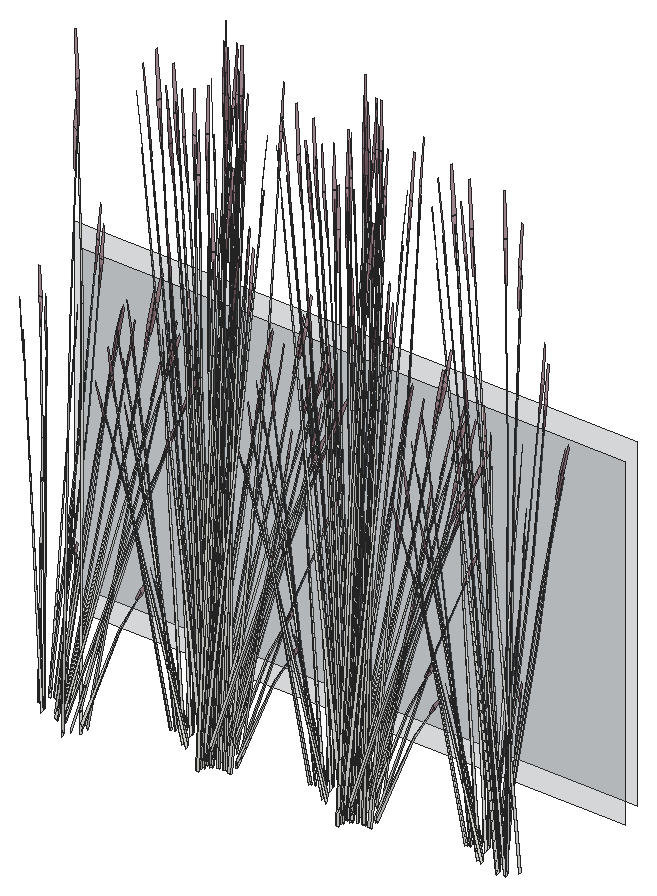
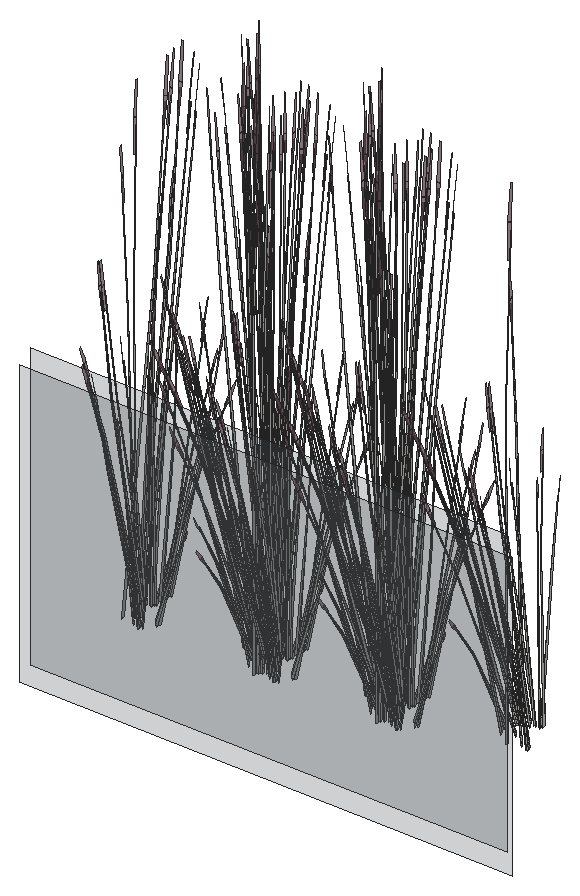
# SketchUp Ruby script. Lengths in inches.
U = 1.inch
M = Sketchup.active_model
def pt(a) = Geom::Point3d.new(a.map { |v| v * U })
def face(e, loops, mat)
  f = e.add_face(loops[0].map { |a| pt(a) })
  loops[1..].each { |l| e.add_face(l.map { |a| pt(a) }).erase! }
  f.material = f.back_material = mat if mat
  f
end
# faces: each face lists its corners as indices into pts; further lists are holes
def faces(e, pts, list, mat = nil) = list.each { |f| face(e, (f[0].is_a?(Array) ? f : [f]).map { |l| l.map { |i| pts[i] } }, mat) }
# xy, xz, yz: faces in a plane at the given z, y or x. An outline is a flat list of corners, or four numbers for a rectangle; further outlines are holes
def ring(l) = l.size == 4 ? [[l[0], l[1]], [l[2], l[1]], [l[2], l[3]], [l[0], l[3]]] : l.each_slice(2).to_a
def flat(e, list, mat, &to3) = list.each { |f| face(e, (f[0].is_a?(Array) ? f : [f]).map { |l| ring(l).map { |u, v| to3.(u, v) } }, mat) }
def xy(e, z, list, mat = nil) = flat(e, list, mat) { |x, y| [x, y, z] }
def xz(e, y, list, mat = nil) = flat(e, list, mat) { |x, z| [x, y, z] }
def yz(e, x, list, mat = nil) = flat(e, list, mat) { |y, z| [x, y, z] }
def lines(e, pts, list) = list.each { |a, b| e.add_line(pt(pts[a]), pt(pts[b])) }
# prism: a flat outline (further loops are holes) pulled along v
def prism(e, loops, v, mat = nil)
  f = face(e, loops, mat); d = Geom::Vector3d.new(v.map { |x| x * U })
  f.pushpull(f.normal.samedirection?(d) ? d.length : -d.length)
end
def box(e, o, s, mat = nil) = prism(e, [[o, [o[0] + s[0], o[1], o[2]], [o[0] + s[0], o[1] + s[1], o[2]], [o[0], o[1] + s[1], o[2]]]], [0, 0, s[2]], mat)
def at(x, y, z, deg = 0) = Geom::Transformation.translation(pt([x, y, z])) * Geom::Transformation.rotation(ORIGIN, Z_AXIS, deg.degrees)
def axes(o, x, y, z) = Geom::Transformation.new([*x, 0, *y, 0, *z, 0, *pt(o).to_a, 1])
def part(name) = M.definitions.add(name)
# library, detail: a bought-in or finely detailed component or shape, given as its bounding box
def library(name, o, s) = part(name).tap { |d| box(d.entities, o, s) }
def detail(e, o, s) = box(e.add_group.entities, o, s)
def put(e, d, t, mat = nil) = e.add_instance(d, t).tap { |i| i.material = mat if mat }
def group(e, t, mat = nil) = e.add_group.tap { |g| g.transformation = t; g.material = mat if mat }.entities
root = M.entities
M.materials.add("Glass_Basic_01").color = [105, 113, 122]
M.materials["Glass_Basic_01"].alpha = 0.25
M.materials.add("LightPink_Translucent").color = [144, 107, 117]
M.materials["LightPink_Translucent"].alpha = 0.75
c1 = part("blade")
p = [[2.15,0.21,22],[0,0.17,0],[0.09,0.45,0],[2.18,0.31,22],[2.29,0.31,22],[0.38,0.45,0],
  [2.48,0.24,33],[2.49,0.24,33],[2.48,0.22,33]]
faces(c1.entities,p,[[0,1,2,3],[4,5,2,3],[6,3,4,7],[8,0,3,6]])
c2 = part("seeds")
p = [[0.3,-0.1,1.38],[-0.01,-0.03,1.59],[-0.01,-0.03,0.03],[0.14,-0.07,-0.07],[0.29,-0.03,3],[0.15,0.01,3.11]]
faces(c2.entities,p,[[0,1,2,3],[1,0,4,5]],"LightPink_Translucent")
c3 = part("blade with seeds")
put(c3.entities,c1,at(0,0,0))
put(c3.entities,c2,axes([2.4,0.25,30.99],[1.5799,-0.05474,1.17369],[-0.12525,1.92788,0.29478],[-0.07173,-0.02425,1.56792]))
xz(root,474,[[218,398,271.49,430]],"Glass_Basic_01")
xz(root,477,[[215,398,270.25,430]],"Glass_Basic_01")
put(root,c3,axes([227.49,457.1,399.875],[0.1255,-0.16547,1.71376],[0.31687,0.44665,0.13857],[-0.21734,0.2034,0.73262]))
put(root,c3,axes([227.39,457.51,399.875],[0.09355,-0.18511,1.71376],[0.39247,0.38307,0.13857],[-0.17705,0.23875,0.73262]))
put(root,c3,axes([227.09,457.59,400.68],[0.12908,0.49174,-0.51099],[-0.48882,0.08602,-0.3958],[-0.14008,0.13208,0.97773]))
put(root,c3,axes([227.34,459.37,398.59],[0.15856,-0.08496,1.43002],[0.39147,0.25616,-0.30754],[-0.11652,0.22165,0.61141]))
put(root,c3,axes([227.5,458.56,400.53],[-0.33997,0.28354,-0.35414],[-0.32182,-0.32376,0.4572],[-0.04897,0.1645,0.87481]))
put(root,c3,axes([227.73,458.26,401.34],[-0.01307,0.49815,-0.7886],[-0.55054,-0.03346,0.09517],[-0.0581,0.21104,1.11556]))
put(root,c3,axes([227.72,459.66,398.77],[-0.013,-0.32022,1.1486],[0.32493,0.22839,0.84392],[-0.0639,0.15263,0.25299]))
put(root,c3,axes([227.54,458.96,399.36],[0.01104,-0.27801,1.54345],[0.49652,0.14685,0.21329],[-0.04302,0.2963,0.72882]))
put(root,c3,axes([227.84,458.42,401],[0.35968,0.36185,-0.5672],[-0.37996,0.3169,-0.43934],[-0.05473,0.18385,1.08528]))
put(root,c3,axes([229.96,456.59,398.84],[-0.01373,-0.50706,1.41272],[0.62119,0.13144,0.59816],[-0.14692,0.27746,1.3335]))
put(root,c3,axes([227.45,458.96,398.82],[0.45645,-0.09537,0.06507],[0.10494,0.38421,-0.86304],[-0.02894,0.19449,0.7736]))
put(root,c3,axes([228.25,457.9,399.875],[-0.0123,-0.2067,1.71376],[0.53301,0.13712,0.13857],[-0.03297,0.29456,0.73262]))
put(root,c3,axes([230.23,458.73,398.375],[0.31414,0.53965,0],[-0.52557,0.30095,-0.51607],[-0.1197,0.06854,1.63711]))
put(root,c3,axes([228.68,459.06,400.53],[-0.15148,0.41415,-0.35414],[-0.44193,-0.12079,0.4572],[0.04052,0.16674,0.87481]))
put(root,c3,axes([228.73,458.68,400.98],[0.23981,0.43789,-0.71045],[-0.49365,0.24404,0.08574],[0.05608,0.21158,1.00501]))
put(root,c3,axes([228.91,458.77,400.68],[0.49392,0.135,-0.51099],[-0.1693,0.46287,-0.3958],[0.04529,0.18636,0.97773]))
put(root,c3,axes([229.1875,457.82,399.875],[-0.11485,-0.17291,1.71376],[0.53072,-0.14557,0.13857],[0.11995,0.27145,0.73262]))
put(root,c3,axes([230.65,458.33,398.77],[-0.2829,-0.15485,1.1486],[0.36529,-0.15734,0.84392],[0.09853,0.13328,0.25299]))
put(root,c3,axes([229.64,458.17,398.59],[0.00887,-0.17852,1.43002],[0.42372,-0.19941,-0.30754],[0.1308,0.21367,0.61141]))
put(root,c3,axes([230.69,459.04,398.67],[-0.3222,-0.01689,1.0506],[0.21278,-0.35872,0.58006],[0.12729,0.12745,0.8241]))
put(root,c3,axes([230.01,458.55,400.68],[0.4958,-0.12802,-0.51099],[0.08673,0.48481,-0.3958],[0.13317,0.13893,0.97773]))
put(root,c3,axes([238.09,461,399.875],[0.17434,-0.11391,1.71376],[0.14677,0.52637,0.13857],[-0.27369,0.11897,0.73262]))
put(root,c3,axes([237.55,461.89,398.59],[0.17462,0.04421,1.43002],[0.11254,0.45156,-0.30754],[-0.23719,0.08453,0.61141]))
put(root,c3,axes([239.1,460.45,399.34],[0.14282,-0.0779,1.77064],[0.04925,0.54394,0.13857],[-0.30935,0.07218,0.63284]))
put(root,c3,axes([229.96,457.28,399.875],[-0.18664,-0.09279,1.71376],[0.38624,-0.38925,0.13857],[0.24072,0.1756,0.73262]))
put(root,c3,axes([237.82,460.52,400.53],[-0.41757,-0.15024,-0.35414],[0.12179,-0.4383,0.4572],[-0.16812,0.04019,0.87481]))
put(root,c3,axes([238.11,460.74,400.68],[-0.13612,0.48987,-0.51099],[-0.46669,-0.16791,-0.3958],[-0.1879,0.04492,0.97773]))
put(root,c3,axes([237.1875,462.84,398.77],[0.2094,-0.24408,1.1486],[0.08263,0.38639,0.84392],[-0.15132,0.06919,0.25299]))
put(root,c3,axes([238.73,461.35,399.875],[0.1255,-0.16547,1.71376],[0.31687,0.44665,0.13857],[-0.21734,0.2034,0.73262]))
put(root,c3,axes([237.98,461.78,400.53],[-0.43736,0.07697,-0.35414],[-0.11549,-0.43998,0.4572],[-0.12533,0.11818,0.87481]))
put(root,c3,axes([238.64,461.76,399.875],[0.09355,-0.18511,1.71376],[0.39247,0.38307,0.13857],[-0.17705,0.23875,0.73262]))
put(root,c3,axes([238.34,461.83,400.68],[0.12908,0.49174,-0.51099],[-0.48882,0.08602,-0.3958],[-0.14008,0.13208,0.97773]))
put(root,c3,axes([239.16,462.84,398.375],[-0.31414,0.53965,0],[-0.52557,-0.30095,-0.51607],[-0.1197,-0.06854,1.63711]))
put(root,c3,axes([238.58,463.62,398.59],[0.15856,-0.08496,1.43002],[0.39147,0.25616,-0.30754],[-0.11652,0.22165,0.61141]))
put(root,c3,axes([240.15,461.5625,398.67],[-0.5073,0.35754,-0.29095],[-0.33735,-0.5052,-0.50002],[-0.12516,-0.05131,1.59708]))
put(root,c3,axes([238.75,462.8,400.53],[-0.33997,0.28354,-0.35414],[-0.32182,-0.32376,0.4572],[-0.04897,0.1645,0.87481]))
put(root,c3,axes([240.72,461.73,398.46],[-0.49063,-0.43346,-0.25192],[0.41285,-0.48673,0.5513],[-0.13212,0.05071,1.68216]))
put(root,c3,axes([238.97,462.5,401.34],[-0.01307,0.49815,-0.7886],[-0.55054,-0.03346,0.09517],[-0.0581,0.21104,1.11556]))
put(root,c3,axes([238.96,463.9,398.77],[-0.013,-0.32022,1.1486],[0.32493,0.22839,0.84392],[-0.0639,0.15263,0.25299]))
put(root,c3,axes([239.43,462.56,398.48],[0.47024,0.26927,0.49651],[-0.28107,0.48284,0],[-0.1071,-0.06133,1.57504]))
put(root,c3,axes([238.79,463.2,399.36],[0.01104,-0.27801,1.54345],[0.49652,0.14685,0.21329],[-0.04302,0.2963,0.72882]))
put(root,c3,axes([240.1,461.72,398.62],[-0.09693,0.48062,0.1448],[-0.47357,-0.08343,-0.41347],[-0.08619,-0.04935,1.26744]))
put(root,c3,axes([241.08,462.91,398.19],[-0.31023,-0.54153,-0.05142],[0.52557,-0.30095,0.51607],[-0.12951,0.05156,1.6363]))
put(root,c3,axes([239.08,462.67,401],[0.35968,0.36185,-0.5672],[-0.37996,0.3169,-0.43934],[-0.05473,0.18385,1.08528]))
put(root,c3,axes([241.2,460.84,398.84],[-0.01373,-0.50706,1.41272],[0.62119,0.13144,0.59816],[-0.14692,0.27746,1.3335]))
put(root,c3,axes([238.69,463.21,398.82],[0.45645,-0.09537,0.06507],[0.10494,0.38421,-0.86304],[-0.02894,0.19449,0.7736]))
put(root,c3,axes([239.49,462.15,399.875],[-0.0123,-0.2067,1.71376],[0.53301,0.13712,0.13857],[-0.03297,0.29456,0.73262]))
put(root,c3,axes([239.94,461.26,398.36],[0.63506,0.11347,0.45755],[-0.12924,0.64083,0.17955],[-0.09281,-0.06188,1.58856]))
put(root,c3,axes([239.6,462.28,398.47],[0.53992,-0.14294,0.17642],[0.13332,0.53195,0.35086],[-0.04815,-0.07751,1.60407]))
put(root,c3,axes([240.3,462.37,398.2],[-0.50654,-0.24178,0],[0.24378,-0.50239,0],[0,0,1.62707]))
put(root,c3,axes([241.47,462.97,398.375],[0.31414,0.53965,0],[-0.52557,0.30095,-0.51607],[-0.1197,0.06854,1.63711]))
put(root,c3,axes([241.21,462.3125,398.47],[0.14515,-0.53522,0.17642],[0.53115,0.15146,0.35086],[-0.09175,0.00261,1.60407]))
put(root,c3,axes([240.97,461.6,398.62],[0.37121,0.32357,0.1448],[-0.30963,0.36505,-0.41347],[-0.08619,0.04935,1.26744]))
put(root,c3,axes([240.96,461.37,398.72],[0.54562,-0.03324,0.44739],[0.04934,0.55185,-0.21531],[-0.09768,0.05593,1.43643]))
put(root,c3,axes([241.09,462.63,398.33],[0.62903,0.17504,0.30756],[-0.15737,0.62568,-0.36492],[-0.10411,0.07831,1.64885]))
put(root,c3,axes([241.36,462.6,398.48],[0.47024,-0.26927,0.49651],[0.28107,0.48284,0],[-0.1071,0.06133,1.57504]))
put(root,c3,axes([240.41,462.16,398.2],[-0.16394,-0.4643,0],[0.46814,-0.1626,0],[0,0,1.54371]))
put(root,c3,axes([239.93,463.3,400.53],[-0.15148,0.41415,-0.35414],[-0.44193,-0.12079,0.4572],[0.04052,0.16674,0.87481]))
put(root,c3,axes([242.04,460.95,398.47],[-0.39477,-0.39228,0.17642],[0.39783,-0.38049,0.35086],[-0.0436,0.08011,1.60407]))
put(root,c3,axes([240.99,460.97,398.29],[0,0.62282,-0.05637],[-0.62828,0,0],[0,0.01957,1.79368]))
put(root,c3,axes([240.69,462.18,398.29],[0.21845,0.61869,-0.06012],[-0.62418,0.21679,0],[0.00763,0.02161,1.72173]))
put(root,c3,axes([239.97,462.93,400.98],[0.23981,0.43789,-0.71045],[-0.49365,0.24404,0.08574],[0.05608,0.21158,1.00501]))
put(root,c3,axes([242.5,461.36,398.2],[-0.62797,-0.00431,-0.04976],[0,-0.6019,0.49943],[-0.01973,0.13702,1.58352]))
put(root,c3,axes([241.26,459.55,398.47],[-0.53992,0.14294,0.17642],[-0.13332,-0.53195,0.35086],[0.04815,0.07751,1.60407]))
put(root,c3,axes([241.09,461.1,398.21],[0.35073,0.34786,0],[-0.35073,0.34786,0],[0,0,1.69266]))
put(root,c3,axes([241.08,460.69,398.72],[0.24378,-0.48527,0.44739],[0.50654,0.23354,-0.21531],[0,0.11186,1.43643]))
put(root,c3,axes([240.875,462.38,398.2],[0.50654,0.24178,0],[-0.24378,0.50239,0],[0,0,1.74954]))
put(root,c3,axes([240.15,463.02,400.68],[0.49392,0.135,-0.51099],[-0.1693,0.46287,-0.3958],[0.04529,0.18636,0.97773]))
put(root,c3,axes([240.92,460.58,398.38],[-0.63506,-0.11347,0.49198],[0.12924,-0.64083,0.19306],[0.09281,0.06188,1.70813]))
put(root,c3,axes([241.1,460.86,398.21],[0.56215,0,0],[0,0.55754,0],[0,0,1.78407]))
put(root,c3,axes([240.5625,460.25,398.72],[-0.30184,-0.45202,0.44739],[0.45719,-0.31831,-0.21531],[0.09768,0.05593,1.43643]))
put(root,c3,axes([241.3,460.8,398.62],[0.46814,-0.15705,0.1448],[0.16394,0.44848,-0.41347],[0,0.0987,1.26744]))
put(root,c3,axes([242.36,460.96,398.48],[0,-0.53854,0.49651],[0.56215,0,0],[0,0.12266,1.57504]))
put(root,c3,axes([240.43,462.0625,399.875],[-0.11485,-0.17291,1.71376],[0.53072,-0.14557,0.13857],[0.11995,0.27145,0.73262]))
put(root,c3,axes([240.76,460.12,398.62],[0.09693,-0.48062,0.1448],[0.47357,0.08343,-0.41347],[0.08619,0.04935,1.26744]))
put(root,c3,axes([241.03,462.09,398.18],[0.5275,-0.18273,-0.19198],[0.18536,0.52636,0.00008],[0.05823,-0.0202,1.73897]))
put(root,c3,axes([241.89,462.58,398.77],[-0.2829,-0.15485,1.1486],[0.36529,-0.15734,0.84392],[0.09853,0.13328,0.25299]))
put(root,c3,axes([240.88,462.41,398.59],[0.00887,-0.17852,1.43002],[0.42372,-0.19941,-0.30754],[0.1308,0.21367,0.61141]))
put(root,c3,axes([242.75,461.05,398.375],[0.62828,0,0],[0,0.6019,-0.51607],[0,0.13709,1.63711]))
put(root,c3,axes([240.72,460.27,398.67],[0.5073,-0.35754,-0.29095],[0.33735,0.5052,-0.50002],[0.12516,0.05131,1.59708]))
put(root,c3,axes([241.9375,463.28,398.67],[-0.3222,-0.01689,1.0506],[0.21278,-0.35872,0.58006],[0.12729,0.12745,0.8241]))
put(root,c3,axes([241.25,462.79,400.68],[0.4958,-0.12802,-0.51099],[0.08673,0.48481,-0.3958],[0.13317,0.13893,0.97773]))
put(root,c3,axes([243.08,462.4375,399.93],[-0.09617,-0.45271,-0.03492],[0.45453,-0.10408,-0.15832],[0.09492,0.0287,0.52218]))
put(root,c3,axes([241.2,461.52,399.875],[-0.18664,-0.09279,1.71376],[0.38624,-0.38925,0.13857],[0.24072,0.1756,0.73262]))
put(root,c3,axes([242.23,462.39,400.53],[0.28589,0.33718,-0.35414],[-0.32644,0.31919,0.4572],[0.16586,0.04856,0.87481]))
put(root,c3,axes([243.62,461.31,398.77],[-0.31044,0.08891,1.1486],[0.14613,-0.36744,0.84392],[0.16469,0.02514,0.25299]))
put(root,c3,axes([242.73,461.22,400.53],[0.41757,0.15024,-0.35414],[-0.12179,0.4383,0.4572],[0.16812,-0.04019,0.87481]))
put(root,c3,axes([241.93,462.16,400.98],[0.50227,0.01297,-0.71045],[-0.03373,0.54602,0.08574],[0.21278,0.05762,1.00501]))
put(root,c3,axes([241.59,460.67,399.875],[-0.20841,0.0122,1.71376],[0.13825,-0.52864,0.13857],[0.297,0.0327,0.73262]))
put(root,c3,axes([251.8,461,399.875],[0.17434,-0.11391,1.71376],[0.14677,0.52637,0.13857],[-0.27369,0.11897,0.73262]))
put(root,c3,axes([251.26,461.89,398.59],[0.17462,0.04421,1.43002],[0.11254,0.45156,-0.30754],[-0.23719,0.08453,0.61141]))
put(root,c3,axes([243.04,461.9,398.59],[-0.12101,-0.13245,1.43002],[0.15744,-0.43816,-0.30754],[0.24483,0.05936,0.61141]))
put(root,c3,axes([252.8,460.45,399.34],[0.14282,-0.0779,1.77064],[0.04925,0.54394,0.13857],[-0.30935,0.07218,0.63284]))
put(root,c3,axes([251.53,460.52,400.53],[-0.41757,-0.15024,-0.35414],[0.12179,-0.4383,0.4572],[-0.16812,0.04019,0.87481]))
put(root,c3,axes([251.82,460.74,400.68],[-0.13612,0.48987,-0.51099],[-0.46669,-0.16791,-0.3958],[-0.1879,0.04492,0.97773]))
put(root,c3,axes([250.89,462.84,398.77],[0.2094,-0.24408,1.1486],[0.08263,0.38639,0.84392],[-0.15132,0.06919,0.25299]))
put(root,c3,axes([252.44,461.35,399.875],[0.1255,-0.16547,1.71376],[0.31687,0.44665,0.13857],[-0.21734,0.2034,0.73262]))
put(root,c3,axes([251.68,461.78,400.53],[-0.43736,0.07697,-0.35414],[-0.11549,-0.43998,0.4572],[-0.12533,0.11818,0.87481]))
put(root,c3,axes([252.35,461.76,399.875],[0.09355,-0.18511,1.71376],[0.39247,0.38307,0.13857],[-0.17705,0.23875,0.73262]))
put(root,c3,axes([252.05,461.83,400.68],[0.12908,0.49174,-0.51099],[-0.48882,0.08602,-0.3958],[-0.14008,0.13208,0.97773]))
put(root,c3,axes([252.86,462.84,398.375],[-0.31414,0.53965,0],[-0.52557,-0.30095,-0.51607],[-0.1197,-0.06854,1.63711]))
put(root,c3,axes([252.29,463.62,398.59],[0.15856,-0.08496,1.43002],[0.39147,0.25616,-0.30754],[-0.11652,0.22165,0.61141]))
put(root,c3,axes([253.86,461.5625,398.67],[-0.5073,0.35754,-0.29095],[-0.33735,-0.5052,-0.50002],[-0.12516,-0.05131,1.59708]))
put(root,c3,axes([252.45,462.8,400.53],[-0.33997,0.28354,-0.35414],[-0.32182,-0.32376,0.4572],[-0.04897,0.1645,0.87481]))
put(root,c3,axes([254.43,461.73,398.46],[-0.49063,-0.43346,-0.25192],[0.41285,-0.48673,0.5513],[-0.13212,0.05071,1.68216]))
put(root,c3,axes([252.68,462.5,401.34],[-0.01307,0.49815,-0.7886],[-0.55054,-0.03346,0.09517],[-0.0581,0.21104,1.11556]))
put(root,c3,axes([252.67,463.9,398.77],[-0.013,-0.32022,1.1486],[0.32493,0.22839,0.84392],[-0.0639,0.15263,0.25299]))
put(root,c3,axes([253.14,462.56,398.48],[0.47024,0.26927,0.49651],[-0.28107,0.48284,0],[-0.1071,-0.06133,1.57504]))
put(root,c3,axes([252.5,463.2,399.36],[0.01104,-0.27801,1.54345],[0.49652,0.14685,0.21329],[-0.04302,0.2963,0.72882]))
put(root,c3,axes([253.81,461.72,398.62],[-0.09693,0.48062,0.1448],[-0.47357,-0.08343,-0.41347],[-0.08619,-0.04935,1.26744]))
put(root,c3,axes([254.78,462.91,398.19],[-0.31023,-0.54153,-0.05142],[0.52557,-0.30095,0.51607],[-0.12951,0.05156,1.6363]))
put(root,c3,axes([252.79,462.67,401],[0.35968,0.36185,-0.5672],[-0.37996,0.3169,-0.43934],[-0.05473,0.18385,1.08528]))
put(root,c3,axes([254.91,460.84,398.84],[-0.01373,-0.50706,1.41272],[0.62119,0.13144,0.59816],[-0.14692,0.27746,1.3335]))
put(root,c3,axes([252.4,463.21,398.82],[0.45645,-0.09537,0.06507],[0.10494,0.38421,-0.86304],[-0.02894,0.19449,0.7736]))
put(root,c3,axes([254.5625,461.48,398.67],[0.05855,0.61451,-0.29095],[-0.60981,0.03716,-0.50002],[-0.10738,0.08185,1.59708]))
put(root,c3,axes([253.2,462.15,399.875],[-0.0123,-0.2067,1.71376],[0.53301,0.13712,0.13857],[-0.03297,0.29456,0.73262]))
put(root,c3,axes([253.65,461.26,398.36],[0.63506,0.11347,0.45755],[-0.12924,0.64083,0.17955],[-0.09281,-0.06188,1.58856]))
put(root,c3,axes([253.3125,462.28,398.47],[0.53992,-0.14294,0.17642],[0.13332,0.53195,0.35086],[-0.04815,-0.07751,1.60407]))
put(root,c3,axes([254.01,462.37,398.2],[-0.50654,-0.24178,0],[0.24378,-0.50239,0],[0,0,1.62707]))
put(root,c3,axes([255.18,462.97,398.375],[0.31414,0.53965,0],[-0.52557,0.30095,-0.51607],[-0.1197,0.06854,1.63711]))
put(root,c3,axes([254.92,462.3125,398.47],[0.14515,-0.53522,0.17642],[0.53115,0.15146,0.35086],[-0.09175,0.00261,1.60407]))
put(root,c3,axes([254.67,461.6,398.62],[0.37121,0.32357,0.1448],[-0.30963,0.36505,-0.41347],[-0.08619,0.04935,1.26744]))
put(root,c3,axes([254.66,461.37,398.72],[0.54562,-0.03324,0.44739],[0.04934,0.55185,-0.21531],[-0.09768,0.05593,1.43643]))
put(root,c3,axes([254.8,462.63,398.33],[0.62903,0.17504,0.30756],[-0.15737,0.62568,-0.36492],[-0.10411,0.07831,1.64885]))
put(root,c3,axes([255.07,462.6,398.48],[0.47024,-0.26927,0.49651],[0.28107,0.48284,0],[-0.1071,0.06133,1.57504]))
put(root,c3,axes([254.12,462.16,398.2],[-0.16394,-0.4643,0],[0.46814,-0.1626,0],[0,0,1.54371]))
put(root,c3,axes([253.63,463.3,400.53],[-0.15148,0.41415,-0.35414],[-0.44193,-0.12079,0.4572],[0.04052,0.16674,0.87481]))
put(root,c3,axes([255.75,460.95,398.47],[-0.39477,-0.39228,0.17642],[0.39783,-0.38049,0.35086],[-0.0436,0.08011,1.60407]))
put(root,c3,axes([254.7,460.97,398.29],[0,0.62282,-0.05637],[-0.62828,0,0],[0,0.01957,1.79368]))
put(root,c3,axes([254.4,462.18,398.29],[0.21845,0.61869,-0.06012],[-0.62418,0.21679,0],[0.00763,0.02161,1.72173]))
put(root,c3,axes([253.68,462.93,400.98],[0.23981,0.43789,-0.71045],[-0.49365,0.24404,0.08574],[0.05608,0.21158,1.00501]))
put(root,c3,axes([256.2,461.36,398.2],[-0.62797,-0.00431,-0.04976],[0,-0.6019,0.49943],[-0.01973,0.13702,1.58352]))
put(root,c3,axes([254.97,459.55,398.47],[-0.53992,0.14294,0.17642],[-0.13332,-0.53195,0.35086],[0.04815,0.07751,1.60407]))
put(root,c3,axes([254.8,461.1,398.21],[0.35073,0.34786,0],[-0.35073,0.34786,0],[0,0,1.69266]))
put(root,c3,axes([254.79,460.69,398.72],[0.24378,-0.48527,0.44739],[0.50654,0.23354,-0.21531],[0,0.11186,1.43643]))
put(root,c3,axes([254.58,462.38,398.2],[0.50654,0.24178,0],[-0.24378,0.50239,0],[0,0,1.74954]))
put(root,c3,axes([253.86,463.02,400.68],[0.49392,0.135,-0.51099],[-0.1693,0.46287,-0.3958],[0.04529,0.18636,0.97773]))
put(root,c3,axes([254.63,460.58,398.38],[-0.63506,-0.11347,0.49198],[0.12924,-0.64083,0.19306],[0.09281,0.06188,1.70813]))
put(root,c3,axes([254.81,460.86,398.21],[0.56215,0,0],[0,0.55754,0],[0,0,1.78407]))
put(root,c3,axes([254.27,460.25,398.72],[-0.30184,-0.45202,0.44739],[0.45719,-0.31831,-0.21531],[0.09768,0.05593,1.43643]))
put(root,c3,axes([255,460.8,398.62],[0.46814,-0.15705,0.1448],[0.16394,0.44848,-0.41347],[0,0.0987,1.26744]))
put(root,c3,axes([254.84,460.84,398.67],[0.56585,0.25696,-0.29095],[-0.27246,0.54236,-0.50002],[0.01778,0.13316,1.59708]))
put(root,c3,axes([256.07,460.96,398.48],[0,-0.53854,0.49651],[0.56215,0,0],[0,0.12266,1.57504]))
put(root,c3,axes([254.14,462.0625,399.875],[-0.11485,-0.17291,1.71376],[0.53072,-0.14557,0.13857],[0.11995,0.27145,0.73262]))
put(root,c3,axes([254.47,460.12,398.62],[0.09693,-0.48062,0.1448],[0.47357,0.08343,-0.41347],[0.08619,0.04935,1.26744]))
put(root,c3,axes([254.73,462.09,398.18],[0.5275,-0.18273,-0.19198],[0.18536,0.52636,0.00008],[0.05823,-0.0202,1.73897]))
put(root,c3,axes([255.6,462.58,398.77],[-0.2829,-0.15485,1.1486],[0.36529,-0.15734,0.84392],[0.09853,0.13328,0.25299]))
put(root,c3,axes([254.59,462.41,398.59],[0.00887,-0.17852,1.43002],[0.42372,-0.19941,-0.30754],[0.1308,0.21367,0.61141]))
put(root,c3,axes([256.45,461.05,398.375],[0.62828,0,0],[0,0.6019,-0.51607],[0,0.13709,1.63711]))
put(root,c3,axes([254.42,460.27,398.67],[0.5073,-0.35754,-0.29095],[0.33735,0.5052,-0.50002],[0.12516,0.05131,1.59708]))
put(root,c3,axes([255.64,463.28,398.67],[-0.3222,-0.01689,1.0506],[0.21278,-0.35872,0.58006],[0.12729,0.12745,0.8241]))
put(root,c3,axes([254.96,462.79,400.68],[0.4958,-0.12802,-0.51099],[0.08673,0.48481,-0.3958],[0.13317,0.13893,0.97773]))
put(root,c3,axes([256.79,462.4375,399.93],[-0.09617,-0.45271,-0.03492],[0.45453,-0.10408,-0.15832],[0.09492,0.0287,0.52218]))
put(root,c3,axes([254.91,461.52,399.875],[-0.18664,-0.09279,1.71376],[0.38624,-0.38925,0.13857],[0.24072,0.1756,0.73262]))
put(root,c3,axes([255.94,462.39,400.53],[0.28589,0.33718,-0.35414],[-0.32644,0.31919,0.4572],[0.16586,0.04856,0.87481]))
put(root,c3,axes([257.33,461.31,398.77],[-0.31044,0.08891,1.1486],[0.14613,-0.36744,0.84392],[0.16469,0.02514,0.25299]))
put(root,c3,axes([256.44,461.22,400.53],[0.41757,0.15024,-0.35414],[-0.12179,0.4383,0.4572],[0.16812,-0.04019,0.87481]))
put(root,c3,axes([255.63,462.16,400.98],[0.50227,0.01297,-0.71045],[-0.03373,0.54602,0.08574],[0.21278,0.05762,1.00501]))
put(root,c3,axes([255.3,460.67,399.875],[-0.20841,0.0122,1.71376],[0.13825,-0.52864,0.13857],[0.297,0.0327,0.73262]))
put(root,c3,axes([256.74,461.9,398.59],[-0.12101,-0.13245,1.43002],[0.15744,-0.43816,-0.30754],[0.24483,0.05936,0.61141]))
put(root,c3,axes([267.05,461,399.875],[0.17434,-0.11391,1.71376],[0.14677,0.52637,0.13857],[-0.27369,0.11897,0.73262]))
put(root,c3,axes([266.51,461.89,398.59],[0.17462,0.04421,1.43002],[0.11254,0.45156,-0.30754],[-0.23719,0.08453,0.61141]))
put(root,c3,axes([268.05,460.45,399.34],[0.14282,-0.0779,1.77064],[0.04925,0.54394,0.13857],[-0.30935,0.07218,0.63284]))
put(root,c3,axes([266.78,460.52,400.53],[-0.41757,-0.15024,-0.35414],[0.12179,-0.4383,0.4572],[-0.16812,0.04019,0.87481]))
put(root,c3,axes([267.07,460.74,400.68],[-0.13612,0.48987,-0.51099],[-0.46669,-0.16791,-0.3958],[-0.1879,0.04492,0.97773]))
put(root,c3,axes([266.14,462.84,398.77],[0.2094,-0.24408,1.1486],[0.08263,0.38639,0.84392],[-0.15132,0.06919,0.25299]))
put(root,c3,axes([267.6875,461.35,399.875],[0.1255,-0.16547,1.71376],[0.31687,0.44665,0.13857],[-0.21734,0.2034,0.73262]))
put(root,c3,axes([266.93,461.78,400.53],[-0.43736,0.07697,-0.35414],[-0.11549,-0.43998,0.4572],[-0.12533,0.11818,0.87481]))
put(root,c3,axes([267.59,461.76,399.875],[0.09355,-0.18511,1.71376],[0.39247,0.38307,0.13857],[-0.17705,0.23875,0.73262]))
put(root,c3,axes([267.29,461.83,400.68],[0.12908,0.49174,-0.51099],[-0.48882,0.08602,-0.3958],[-0.14008,0.13208,0.97773]))
put(root,c3,axes([268.11,462.84,398.375],[-0.31414,0.53965,0],[-0.52557,-0.30095,-0.51607],[-0.1197,-0.06854,1.63711]))
put(root,c3,axes([267.54,463.62,398.59],[0.15856,-0.08496,1.43002],[0.39147,0.25616,-0.30754],[-0.11652,0.22165,0.61141]))
put(root,c3,axes([269.11,461.5625,398.67],[-0.5073,0.35754,-0.29095],[-0.33735,-0.5052,-0.50002],[-0.12516,-0.05131,1.59708]))
put(root,c3,axes([267.7,462.8,400.53],[-0.33997,0.28354,-0.35414],[-0.32182,-0.32376,0.4572],[-0.04897,0.1645,0.87481]))
put(root,c3,axes([269.67,461.73,398.46],[-0.49063,-0.43346,-0.25192],[0.41285,-0.48673,0.5513],[-0.13212,0.05071,1.68216]))
put(root,c3,axes([267.93,462.5,401.34],[-0.01307,0.49815,-0.7886],[-0.55054,-0.03346,0.09517],[-0.0581,0.21104,1.11556]))
put(root,c3,axes([267.92,463.9,398.77],[-0.013,-0.32022,1.1486],[0.32493,0.22839,0.84392],[-0.0639,0.15263,0.25299]))
put(root,c3,axes([268.38,462.56,398.48],[0.47024,0.26927,0.49651],[-0.28107,0.48284,0],[-0.1071,-0.06133,1.57504]))
put(root,c3,axes([267.74,463.2,399.36],[0.01104,-0.27801,1.54345],[0.49652,0.14685,0.21329],[-0.04302,0.2963,0.72882]))
put(root,c3,axes([269.06,461.72,398.62],[-0.09693,0.48062,0.1448],[-0.47357,-0.08343,-0.41347],[-0.08619,-0.04935,1.26744]))
put(root,c3,axes([270.03,462.91,398.19],[-0.31023,-0.54153,-0.05142],[0.52557,-0.30095,0.51607],[-0.12951,0.05156,1.6363]))
put(root,c3,axes([268.04,462.67,401],[0.35968,0.36185,-0.5672],[-0.37996,0.3169,-0.43934],[-0.05473,0.18385,1.08528]))
put(root,c3,axes([270.16,460.84,398.84],[-0.01373,-0.50706,1.41272],[0.62119,0.13144,0.59816],[-0.14692,0.27746,1.3335]))
put(root,c3,axes([267.65,463.21,398.82],[0.45645,-0.09537,0.06507],[0.10494,0.38421,-0.86304],[-0.02894,0.19449,0.7736]))
put(root,c3,axes([269.81,461.48,398.67],[0.05855,0.61451,-0.29095],[-0.60981,0.03716,-0.50002],[-0.10738,0.08185,1.59708]))
put(root,c3,axes([268.45,462.15,399.875],[-0.0123,-0.2067,1.71376],[0.53301,0.13712,0.13857],[-0.03297,0.29456,0.73262]))
